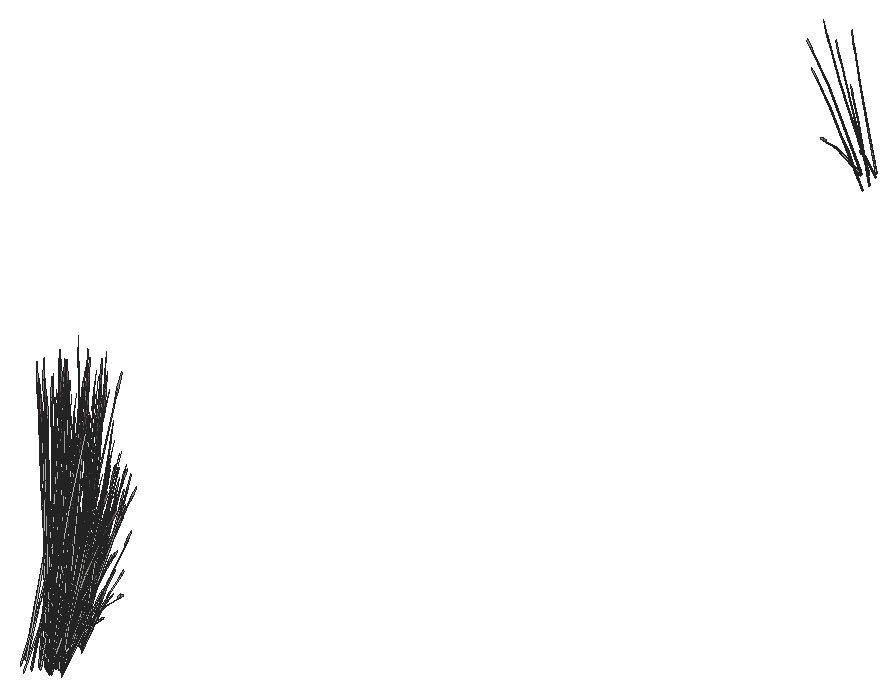
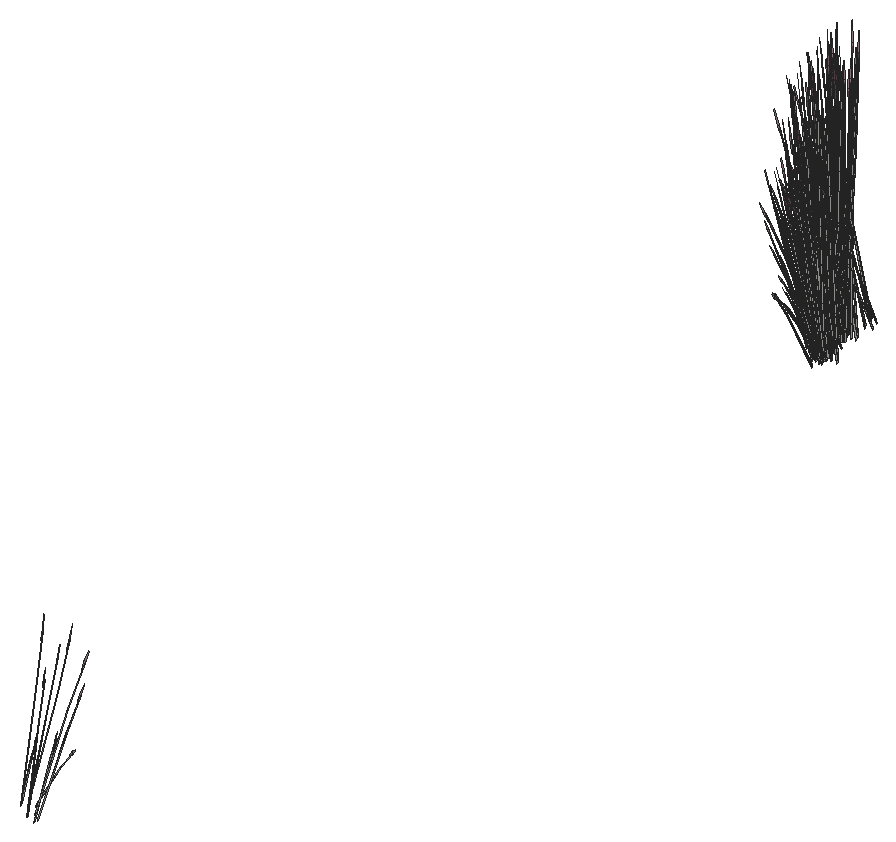
# SketchUp Ruby script. Lengths in inches.
U = 1.inch
M = Sketchup.active_model
def pt(a) = Geom::Point3d.new(a.map { |v| v * U })
def face(e, loops, mat)
  f = e.add_face(loops[0].map { |a| pt(a) })
  loops[1..].each { |l| e.add_face(l.map { |a| pt(a) }).erase! }
  f.material = f.back_material = mat if mat
  f
end
# faces: each face lists its corners as indices into pts; further lists are holes
def faces(e, pts, list, mat = nil) = list.each { |f| face(e, (f[0].is_a?(Array) ? f : [f]).map { |l| l.map { |i| pts[i] } }, mat) }
# xy, xz, yz: faces in a plane at the given z, y or x. An outline is a flat list of corners, or four numbers for a rectangle; further outlines are holes
def ring(l) = l.size == 4 ? [[l[0], l[1]], [l[2], l[1]], [l[2], l[3]], [l[0], l[3]]] : l.each_slice(2).to_a
def flat(e, list, mat, &to3) = list.each { |f| face(e, (f[0].is_a?(Array) ? f : [f]).map { |l| ring(l).map { |u, v| to3.(u, v) } }, mat) }
def xy(e, z, list, mat = nil) = flat(e, list, mat) { |x, y| [x, y, z] }
def xz(e, y, list, mat = nil) = flat(e, list, mat) { |x, z| [x, y, z] }
def yz(e, x, list, mat = nil) = flat(e, list, mat) { |y, z| [x, y, z] }
def lines(e, pts, list) = list.each { |a, b| e.add_line(pt(pts[a]), pt(pts[b])) }
# prism: a flat outline (further loops are holes) pulled along v
def prism(e, loops, v, mat = nil)
  f = face(e, loops, mat); d = Geom::Vector3d.new(v.map { |x| x * U })
  f.pushpull(f.normal.samedirection?(d) ? d.length : -d.length)
end
def box(e, o, s, mat = nil) = prism(e, [[o, [o[0] + s[0], o[1], o[2]], [o[0] + s[0], o[1] + s[1], o[2]], [o[0], o[1] + s[1], o[2]]]], [0, 0, s[2]], mat)
def at(x, y, z, deg = 0) = Geom::Transformation.translation(pt([x, y, z])) * Geom::Transformation.rotation(ORIGIN, Z_AXIS, deg.degrees)
def axes(o, x, y, z) = Geom::Transformation.new([*x, 0, *y, 0, *z, 0, *pt(o).to_a, 1])
def part(name) = M.definitions.add(name)
# library, detail: a bought-in or finely detailed component or shape, given as its bounding box
def library(name, o, s) = part(name).tap { |d| box(d.entities, o, s) }
def detail(e, o, s) = box(e.add_group.entities, o, s)
def put(e, d, t, mat = nil) = e.add_instance(d, t).tap { |i| i.material = mat if mat }
def group(e, t, mat = nil) = e.add_group.tap { |g| g.transformation = t; g.material = mat if mat }.entities
root = M.entities
M.materials.add("LightPink_Translucent").color = [144, 107, 117]
M.materials["LightPink_Translucent"].alpha = 0.75
c1 = part("blade")
p = [[2.15,0.21,22],[0,0.17,0],[0.09,0.45,0],[2.18,0.31,22],[2.29,0.31,22],[0.38,0.45,0],
  [2.48,0.24,33],[2.49,0.24,33],[2.48,0.22,33]]
faces(c1.entities,p,[[0,1,2,3],[4,5,2,3],[6,3,4,7],[8,0,3,6]])
c2 = part("seeds")
p = [[0.3,-0.1,1.38],[-0.01,-0.03,1.59],[-0.01,-0.03,0.03],[0.14,-0.07,-0.07],[0.29,-0.03,3],[0.15,0.01,3.11]]
faces(c2.entities,p,[[0,1,2,3],[1,0,4,5]],"LightPink_Translucent")
c3 = part("blade with seeds")
put(c3.entities,c1,at(0,0,0))
put(c3.entities,c2,axes([2.4,0.25,30.99],[1.5799,-0.05474,1.17369],[-0.12525,1.92788,0.29478],[-0.07173,-0.02425,1.56792]))
put(root,c3,axes([410.29,64.75,-7.64],[0.13855,-0.49442,-0.47583],[0.47502,0.16947,-0.36857],[0.19125,-0.04534,0.91046]))
put(root,c3,axes([409.54,62.74,-9.79],[0.31974,-0.54466,0],[0.53494,0.30375,-0.48057],[0.12184,0.06918,1.52448]))
put(root,c3,axes([407.34,61.09,-9.52],[-0.32795,-0.01705,0.97832],[0.21658,-0.36206,0.54015],[0.12956,0.12863,0.76741]))
put(root,c3,axes([407.69,64.43,-9.8],[0.22235,0.6078,0.42607],[-0.63531,0.21135,0.16719],[0.00776,-0.11168,1.47927]))
put(root,c3,axes([406.39,61,-7.6],[-0.23243,0.34529,0.05988],[-0.331,-0.20103,0.47138],[0.10701,0.1107,0.71878]))
put(root,c3,axes([410.8,64.89,-10.15],[-0.32938,0.06523,1.31842],[-0.05243,-0.51922,0.07547],[0.2307,-0.07859,0.75023]))
put(root,c3,axes([411.4,64.43,-9.89],[-0.31706,-0.34757,-0.06041],[0.34725,-0.31847,-0.27392],[0.09839,-0.02242,0.90349]))
put(root,c3,axes([408.49,64.48,-9.95],[0,-0.62892,0],[0.63949,0,0],[0,0,1.6711]))
put(root,c3,axes([406.49,60.9,-7.59],[-0.50866,0.12474,0.447],[-0.08828,-0.48932,0.36857],[0.11963,0.14421,0.92496]))
put(root,c3,axes([409.27,63.03,-9.69],[-0.47863,-0.27177,0.46235],[0.28609,-0.48733,0],[0.10901,0.0619,1.46668]))
put(root,c3,axes([410.2,64.93,-7.36],[0.44939,-0.24006,-0.66157],[0.25044,0.49415,0.07984],[0.21713,-0.05613,0.93586]))
put(root,c3,axes([408.1875,64.08,-9.8],[-0.42403,0.49328,0.42607],[-0.50377,-0.43543,0.16719],[0.10223,-0.04923,1.47927]))
put(root,c3,axes([406.27,60.21,-9.59],[0.00902,-0.18018,1.33163],[0.43127,-0.20126,-0.28638],[0.13313,0.21566,0.56934]))
put(root,c3,axes([408.65,64.97,-9.86],[-0.47569,-0.46784,-0.05709],[0.47598,-0.46812,0],[-0.01661,-0.01634,1.63492]))
put(root,c3,axes([407.45,63.27,-9.7],[-0.14774,0.54019,0.16428],[-0.54062,-0.15287,0.32672],[0.09339,-0.00263,1.49371]))
put(root,c3,axes([410.14,65.03,-7.3],[-0.42502,-0.15163,0.32977],[0.12396,-0.44238,-0.42575],[0.17112,-0.04056,0.81462]))
put(root,c3,axes([407.23,63.71,-10.52],[-0.50338,0.21762,1.20058],[-0.16022,-0.62439,0.4665],[0.30911,0.01039,1.36553]))
put(root,c3,axes([408.58,63.87,-9.5625],[0.09866,-0.48509,0.13483],[0.48202,0.0842,-0.38503],[0.08772,0.04981,1.18024]))
put(root,c3,axes([411.16,64.55,-10.61],[-0.02673,-0.08252,1.6421],[0.18538,-0.48271,-0.25086],[0.187,-0.00694,0.2797]))
put(root,c3,axes([408.375,64,-9.47],[-0.30722,-0.45622,0.41661],[0.46535,-0.32126,-0.2005],[0.09942,0.05645,1.33761]))
put(root,c3,axes([405.81,59.86,-8.39],[-0.1169,-0.17452,1.59586],[0.54019,-0.14692,0.12904],[0.12209,0.27397,0.68222]))
put(root,c3,axes([407.4,66.06,-9.7],[0.54955,-0.14427,0.16428],[0.1357,0.53689,0.32672],[-0.04901,-0.07823,1.49371]))
put(root,c3,axes([408.53,64.03,-9.52],[0.51635,-0.36087,-0.27094],[0.34336,0.5099,-0.46562],[0.1274,0.05178,1.4872]))
put(root,c3,axes([410.58,64.98,-7.78],[0.42502,0.15163,-0.32977],[-0.12396,0.44238,0.42575],[0.17112,-0.04056,0.81462]))
put(root,c3,axes([409.83,63.07,-10.12],[0.47863,0.27177,-0.46235],[-0.28609,0.48733,0],[0.10901,0.0619,1.46668]))
put(root,c3,axes([408.92,64.62,-9.95],[0.57217,0,0],[0,0.56272,0],[0,0,1.66132]))
put(root,c3,axes([409.09,63.3,-9.7],[-0.54955,0.14427,0.16428],[-0.1357,-0.53689,0.32672],[0.04901,0.07823,1.49371]))
put(root,c3,axes([409.43,64.43,-8.39],[-0.21212,0.01231,1.59586],[0.14072,-0.53355,0.12904],[0.3023,0.033,0.68222]))
put(root,c3,axes([409.7,63.27,-10.11],[0.12013,0.47362,-0.28847],[-0.47712,0.13449,0.28847],[0.09619,0.05462,1.29413]))
put(root,c3,axes([410.52,65.17,-7.6],[0.18783,0.37061,0.05988],[-0.34252,0.1814,0.47138],[0.15099,-0.03579,0.71878]))
put(root,c3,axes([408.74,64.33,-9.78],[-0.64638,-0.11452,0.45814],[0.13155,-0.64678,0.17978],[0.09446,0.06245,1.59061]))
put(root,c3,axes([410.49,65.03,-7.59],[-0.14449,0.4956,0.447],[-0.47502,-0.16947,0.36857],[0.1868,-0.02978,0.92496]))
put(root,c3,axes([408.22,65.93,-9.95],[-0.16686,-0.46861,0],[0.47648,-0.16411,0],[0,0,1.4375]))
put(root,c3,axes([408.85,65.86,-9.97],[0.53691,-0.18442,-0.17877],[0.18866,0.53125,0.00007],[0.05927,-0.02038,1.61933]))
put(root,c3,axes([409.03,66.09,-9.7],[0.14774,-0.54019,0.16428],[0.54062,0.15287,0.32672],[-0.09339,0.00263,1.49371]))
put(root,c3,axes([408.91,64.86,-9.9375],[0.35699,0.35109,0],[-0.35699,0.35109,0],[0,0,1.57621]))
put(root,c3,axes([409.88,64.71,-9.7],[-0.40181,-0.39593,0.16428],[0.40492,-0.38402,0.32672],[-0.04438,0.08086,1.49371]))
put(root,c3,axes([409.13,64.11,-10.08],[0.53199,0.08911,-0.58063],[-0.11226,0.54969,-0.15239],[0.15876,0.06661,1.28164]))
put(root,c3,axes([411.49,65.07,-9.42],[-0.31598,0.08973,1.06958],[0.14873,-0.37085,0.78586],[0.16763,0.02538,0.23558]))
put(root,c3,axes([408.11,66.14,-9.95],[-0.51557,-0.24403,0],[0.24813,-0.50705,0],[0,0,1.51513]))
put(root,c3,axes([408.91,64.45,-9.47],[0.24813,-0.48978,0.41661],[0.51557,0.23571,-0.2005],[0,0.1129,1.33761]))
put(root,c3,axes([411.34,66.64,-7.62],[-0.04624,-0.04758,1.65179],[0.10116,-0.51007,-0.15608],[0.18215,-0.03259,0.29231]))
put(root,c3,axes([408.8125,64.73,-9.87],[0,0.62861,-0.05249],[-0.63949,0,0],[0,0.01975,1.67027]))
put(root,c3,axes([408.86,64.28,-9.94],[0.30722,0.45622,-0.41661],[-0.46535,0.32126,0.2005],[0.09942,0.05645,1.33761]))
put(root,c3,axes([410.9375,66.21,-8.34],[-0.09788,-0.45691,-0.03251],[0.46264,-0.10504,-0.14742],[0.09661,0.02897,0.48626]))
put(root,c3,axes([409.74,66.2,-7.3125],[0.02738,-0.55277,-0.11324],[0.51847,0.01511,-0.62851],[0.19968,0.0384,0.95501]))
put(root,c3,axes([410.21,64.72,-9.69],[0,-0.54355,0.46235],[0.57217,0,0],[0,0.1238,1.46668]))
put(root,c3,axes([406.62,70.43,-9.59],[-0.14537,0.11002,1.33163],[-0.43536,-0.19256,-0.28638],[0.0807,-0.23948,0.56934]))
put(root,c3,axes([408.78,65.13,-9.47],[0.55535,-0.03355,0.41661],[0.05022,0.55698,-0.2005],[-0.09942,0.05645,1.33761]))
put(root,c3,axes([409.12,64.5625,-9.5625],[0.47648,-0.15851,0.13483],[0.16686,0.45265,-0.38503],[0,0.09962,1.18024]))
put(root,c3,axes([409.66,65.98,-7.3],[-0.29098,-0.34031,0.32977],[0.33226,-0.32215,-0.42575],[0.16881,0.04902,0.81462]))
put(root,c3,axes([410.89,65.66,-9.59],[-0.12317,-0.13368,1.33163],[0.16025,-0.44223,-0.28638],[0.24919,0.05991,0.56934]))
put(root,c3,axes([408.69,66.15,-9.95],[0.51557,0.24403,0],[-0.24813,0.50705,0],[0,0,1.62917]))
put(root,c3,axes([406.97,71.25,-7.36],[0.01331,-0.50278,-0.66157],[0.56035,0.03377,0.07984],[0.05914,-0.213,0.93586]))
put(root,c3,axes([410.1875,65.87,-7.61],[0.10971,-0.00919,1.62908],[0.30091,-0.42228,-0.25764],[0.19514,0.05574,0.13065]))
put(root,c3,axes([407.75,70.46,-7.61],[-0.00494,-0.10818,1.62908],[-0.41695,-0.31265,-0.25764],[0.06446,-0.18952,0.13065]))
put(root,c3,axes([406.34,70.99,-8.39],[-0.09522,0.18683,1.59586],[-0.39947,-0.38663,0.12904],[0.18021,-0.24097,0.68222]))
put(root,c3,axes([408.79,65.37,-9.5625],[0.37783,0.32657,0.13483],[-0.31516,0.36844,-0.38503],[-0.08772,0.04981,1.18024]))
put(root,c3,axes([409.76,65.93,-7.36],[0.51122,0.01309,-0.66157],[-0.03434,0.5511,0.07984],[0.21658,0.05816,0.93586]))
put(root,c3,axes([406.86,71.08,-7.64],[-0.3661,-0.36521,-0.47583],[0.38674,-0.31985,-0.36857],[0.0557,-0.18556,0.91046]))
put(root,c3,axes([409.1875,66.375,-9.69],[0.47863,-0.27177,0.46235],[0.28609,0.48733,0],[-0.10901,0.0619,1.46668]))
put(root,c3,axes([408.51,65.95,-9.87],[0.22235,0.62444,-0.05599],[-0.63531,0.21881,0],[0.00776,0.02181,1.60327]))
put(root,c3,axes([410.6,64.82,-9.79],[0.63949,0,0],[0,0.60749,-0.48057],[0,0.13836,1.52448]))
put(root,c3,axes([410.34,65.13,-9.95],[-0.63917,-0.00435,-0.04634],[0,-0.60749,0.46507],[-0.02009,0.13829,1.47457]))
put(root,c3,axes([408.96,64.6,-9.52],[0.57594,0.25935,-0.27094],[-0.27732,0.5474,-0.46562],[0.0181,0.1344,1.4872]))
put(root,c3,axes([407.2,70.94,-7.78],[0.34603,-0.28618,-0.32977],[0.32756,0.32677,0.42575],[0.04984,-0.16603,0.81462]))
put(root,c3,axes([410.07,66.16,-7.78],[0.29098,0.34031,-0.32977],[-0.33226,0.32215,0.42575],[0.16881,0.04902,0.81462]))
put(root,c3,axes([410.21,65.22,-10.11],[-0.35699,0.33913,-0.28847],[-0.35699,-0.33913,0.28847],[0,0.10923,1.29413]))
put(root,c3,axes([409.92,66.29,-7.6],[-0.02575,0.41332,0.05988],[-0.38885,-0.01133,0.47138],[0.14895,0.04325,0.71878]))
put(root,c3,axes([408.9,65.01,-9.94],[-0.24813,0.48978,-0.41661],[-0.51557,-0.23571,0.2005],[0,0.1129,1.33761]))
put(root,c3,axes([409.96,66.16,-7.59],[-0.37709,0.35815,0.447],[-0.32522,-0.38035,0.36857],[0.17692,0.06607,0.92496]))
put(root,c3,axes([408.76,66.57,-7.3],[-0.07899,-0.43781,0.32977],[0.45153,-0.11561,-0.42575],[0.12128,0.12546,0.81462]))
put(root,c3,axes([408.91,66.41,-9.83],[0.64025,0.17667,0.2864],[-0.16018,0.63149,-0.33981],[-0.10597,0.07904,1.53541]))
put(root,c3,axes([410.45,65.23,-10.12],[0,0.54355,-0.46235],[-0.57217,0,0],[0,0.1238,1.46668]))
put(root,c3,axes([407.64,70.77,-10.61],[-0.07655,-0.04282,1.6421],[-0.19662,-0.47839,-0.25086],[0.13264,-0.12982,0.2797]))
put(root,c3,axes([409.02,65.29,-8.39],[-0.18996,-0.09365,1.59586],[0.39312,-0.39287,0.12904],[0.24502,0.17723,0.68222]))
put(root,c3,axes([409.0625,64.06,-7.83],[-0.44191,-0.28242,1.28769],[0.46662,-0.43971,0.5556],[0.14258,0.26499,1.24467]))
put(root,c3,axes([407.2,71.06,-7.59],[0.36417,0.37086,0.447],[-0.38674,0.31985,0.36857],[0.06718,-0.174,0.92496]))
put(root,c3,axes([409.73,66.35,-9.42],[-0.28795,-0.15629,1.06958],[0.37181,-0.1588,0.78586],[0.10029,0.13452,0.23558]))
put(root,c3,axes([407.34,71.09,-7.6],[0.42027,0.02533,0.05988],[-0.01152,0.38243,0.47138],[0.04398,-0.14649,0.71878]))
put(root,c3,axes([408.72,66.8,-7.3125],[0.30474,-0.46525,-0.11324],[0.44133,0.26804,-0.62851],[0.15341,0.13145,0.95501]))
put(root,c3,axes([407.02,71.35,-7.3],[-0.34603,0.28618,0.32977],[-0.32756,-0.32677,-0.42575],[0.04984,-0.16603,0.81462]))
put(root,c3,axes([407.63,72.12,-7.36],[0.26714,-0.42887,-0.66157],[0.46811,0.30479,0.07984],[0.1595,-0.15539,0.93586]))
put(root,c3,axes([407.62,71.92,-7.64],[-0.13138,-0.49631,-0.47583],[0.49754,-0.08682,-0.36857],[0.14258,-0.13331,0.91046]))
put(root,c3,axes([409.3,66.75,-9.79],[0.31974,0.54466,0],[-0.53494,0.30375,-0.48057],[-0.12184,0.06918,1.52448]))
put(root,c3,axes([408.32,67.1875,-7.62],[0.00151,-0.06581,1.65179],[0.43826,-0.29033,-0.15608],[0.15223,0.10363,0.29231]))
put(root,c3,axes([409.81,66.94,-10.61],[0.03726,-0.07847,1.6421],[0.46909,-0.23111,-0.25086],[0.14221,0.11962,0.2797]))
put(root,c3,axes([409.1875,65.15,-10.05],[0.18752,0.49766,-0.6445],[-0.54017,0.17923,-0.16915],[0.02073,0.16852,1.42262]))
put(root,c3,axes([407.85,72.28,-7.3125],[-0.47307,-0.29971,-0.11324],[0.27254,-0.43404,-0.62851],[0.13365,-0.15087,0.95501]))
put(root,c3,axes([409.08,66.57,-7.64],[0.50465,-0.12921,-0.47583],[0.08828,0.48932,-0.36857],[0.13555,0.14022,0.91046]))
put(root,c3,axes([407.68,66.64,-7.3],[0.15418,-0.41799,0.32977],[0.44981,0.12192,-0.42575],[0.04124,0.16829,0.81462]))
put(root,c3,axes([409.77,67.07,-9.52],[-0.32795,-0.01705,0.97832],[0.21658,-0.36206,0.54015],[0.12956,0.12863,0.76741]))
put(root,c3,axes([405.18,70.79,-10.12],[0.47863,-0.27177,-0.46235],[0.28609,0.48733,0],[0.10901,-0.0619,1.46668]))
put(root,c3,axes([408.02,71.73,-9.59],[-0.1827,-0.0161,1.33163],[-0.18717,-0.43188,-0.28638],[0.22444,-0.12218,0.56934]))
put(root,c3,axes([409.02,72.15,-7.62],[-0.0668,-0.00413,1.65179],[-0.27738,-0.44233,-0.15608],[0.11139,-0.14544,0.29231]))
put(root,c3,axes([408.83,66.97,-7.6],[-0.23243,0.34529,0.05988],[-0.331,-0.20103,0.47138],[0.10701,0.1107,0.71878]))
put(root,c3,axes([408.28,68.13,-6.74],[0.35341,-0.31182,-0.06041],[0.32382,0.34152,-0.27392],[0.0228,0.09677,0.90349]))
put(root,c3,axes([405.75,71.9,-10.08],[0.34446,-0.40855,-0.58063],[0.42791,0.37046,-0.15239],[0.13803,-0.10191,1.28164]))
put(root,c3,axes([408.93,66.875,-7.59],[-0.50866,0.12474,0.447],[-0.08828,-0.48932,0.36857],[0.11963,0.14421,0.92496]))
put(root,c3,axes([408.23,70.93,-9.42],[-0.17034,0.27669,1.06958],[-0.14642,-0.37174,0.78586],[0.14069,-0.09315,0.23558]))
put(root,c3,axes([408.7,66.1875,-9.59],[0.00902,-0.18018,1.33163],[0.43127,-0.20126,-0.28638],[0.13313,0.21566,0.56934]))
put(root,c3,axes([407.99,71.97,-7.78],[0.44516,-0.07768,-0.32977],[0.11755,0.44407,0.42575],[0.12757,-0.11927,0.81462]))
put(root,c3,axes([407.54,67.02,-7.6],[-0.37684,0.18473,0.05988],[-0.18445,-0.33686,0.47138],[0.03639,0.14849,0.71878]))
put(root,c3,axes([407.53,66.82,-7.3125],[0.50045,-0.25306,-0.11324],[0.24593,0.44915,-0.62851],[0.06603,0.18927,0.95501]))
put(root,c3,axes([405.375,72.375,-9.52],[-0.05959,-0.62022,-0.27094],[0.62068,-0.0375,-0.46562],[0.1093,-0.08261,1.4872]))
put(root,c3,axes([407.67,66.99,-7.28],[-0.50393,-0.1421,0.49617],[0.17232,-0.46717,0.40911],[0.03028,0.18372,1.0267]))
put(root,c3,axes([407.625,72.23,-7.3],[-0.44516,0.07768,0.32977],[-0.11755,-0.44407,-0.42575],[0.12757,-0.11927,0.81462]))
put(root,c3,axes([407.62,66.92,-10.61],[0.08277,-0.02958,1.6421],[0.49786,0.16279,-0.25086],[0.01456,0.18348,0.2797]))
put(root,c3,axes([405.29,71,-10.11],[0.47712,0.13449,-0.28847],[-0.12013,0.47362,0.28847],[0.09619,-0.05462,1.29413]))
put(root,c3,axes([407.96,66.8,-7.64],[0.50273,0.13626,-0.47583],[-0.17232,0.46717,-0.36857],[0.0461,0.18809,0.91046]))
put(root,c3,axes([408.24,65.83,-8.39],[-0.1169,-0.17452,1.59586],[0.54019,-0.14692,0.12904],[0.12209,0.27397,0.68222]))
put(root,c3,axes([408.03,72.16,-7.6],[0.35109,0.22859,0.05988],[-0.2044,0.32553,0.47138],[0.11256,-0.10524,0.71878]))
put(root,c3,axes([407.93,72.07,-7.59],[0.12683,0.50025,0.447],[-0.49754,0.08682,0.36857],[0.14663,-0.11765,0.92496]))
put(root,c3,axes([409.27,72.67,-7.61],[0.07097,-0.08279,1.62908],[-0.09083,-0.50786,-0.25764],[0.17806,-0.09629,0.13065]))
put(root,c3,axes([407.73,67.08,-7.78],[-0.15418,0.41799,-0.32977],[-0.44981,-0.12192,0.42575],[0.04124,0.16829,0.81462]))
put(root,c3,axes([407.77,66.71,-7.36],[0.24409,0.44196,-0.66157],[-0.50245,0.2463,0.07984],[0.05708,0.21354,0.93586]))
put(root,c3,axes([407.41,67.82,-7.61],[0.06483,0.08753,1.62908],[0.52315,0.03439,-0.25764],[0.05261,0.19303,0.13065]))
put(root,c3,axes([407.875,73.44,-7.3125],[-0.25732,-0.49218,-0.11324],[0.45669,-0.24187,-0.62851],[0.19245,-0.06494,0.95501]))
put(root,c3,axes([407.85,73.02,-7.64],[0.13855,-0.49442,-0.47583],[0.47502,0.16947,-0.36857],[0.19125,-0.04534,0.91046]))
put(root,c3,axes([407.1,71.01,-9.79],[0.31974,-0.54466,0],[0.53494,0.30375,-0.48057],[0.12184,0.06918,1.52448]))
put(root,c3,axes([408.36,73.16,-10.15],[-0.32938,0.06523,1.31842],[-0.05243,-0.51922,0.07547],[0.2307,-0.07859,0.75023]))
put(root,c3,axes([408.96,72.7,-9.89],[-0.31706,-0.34757,-0.06041],[0.34725,-0.31847,-0.27392],[0.09839,-0.02242,0.90349]))
put(root,c3,axes([406.82,71.29,-9.69],[-0.47863,-0.27177,0.46235],[0.28609,-0.48733,0],[0.10901,0.0619,1.46668]))
put(root,c3,axes([407.76,73.2,-7.36],[0.44939,-0.24006,-0.66157],[0.25044,0.49415,0.07984],[0.21713,-0.05613,0.93586]))
put(root,c3,axes([407.7,73.3,-7.3],[-0.42502,-0.15163,0.32977],[0.12396,-0.44238,-0.42575],[0.17112,-0.04056,0.81462]))
put(root,c3,axes([404.79,71.97,-10.52],[-0.50338,0.21762,1.20058],[-0.16022,-0.62439,0.4665],[0.30911,0.01039,1.36553]))
put(root,c3,axes([406.14,72.14,-9.5625],[0.09866,-0.48509,0.13483],[0.48202,0.0842,-0.38503],[0.08772,0.04981,1.18024]))
put(root,c3,axes([408.72,72.82,-10.61],[-0.02673,-0.08252,1.6421],[0.18538,-0.48271,-0.25086],[0.187,-0.00694,0.2797]))
put(root,c3,axes([405.93,72.27,-9.47],[-0.30722,-0.45622,0.41661],[0.46535,-0.32126,-0.2005],[0.09942,0.05645,1.33761]))
put(root,c3,axes([406.09,72.3,-9.52],[0.51635,-0.36087,-0.27094],[0.34336,0.5099,-0.46562],[0.1274,0.05178,1.4872]))
put(root,c3,axes([408.14,73.25,-7.78],[0.42502,0.15163,-0.32977],[-0.12396,0.44238,0.42575],[0.17112,-0.04056,0.81462]))
put(root,c3,axes([407.39,71.34,-10.12],[0.47863,0.27177,-0.46235],[-0.28609,0.48733,0],[0.10901,0.0619,1.46668]))
put(root,c3,axes([406.48,72.89,-9.95],[0.57217,0,0],[0,0.56272,0],[0,0,1.66132]))
put(root,c3,axes([406.98,72.7,-8.39],[-0.21212,0.01231,1.59586],[0.14072,-0.53355,0.12904],[0.3023,0.033,0.68222]))
put(root,c3,axes([407.26,71.54,-10.11],[0.12013,0.47362,-0.28847],[-0.47712,0.13449,0.28847],[0.09619,0.05462,1.29413]))
put(root,c3,axes([408.08,73.43,-7.6],[0.18783,0.37061,0.05988],[-0.34252,0.1814,0.47138],[0.15099,-0.03579,0.71878]))
put(root,c3,axes([408.04,73.3,-7.59],[-0.14449,0.4956,0.447],[-0.47502,-0.16947,0.36857],[0.1868,-0.02978,0.92496]))
put(root,c3,axes([406.41,74.13,-9.97],[0.53691,-0.18442,-0.17877],[0.18866,0.53125,0.00007],[0.05927,-0.02038,1.61933]))
put(root,c3,axes([406.69,72.38,-10.08],[0.53199,0.08911,-0.58063],[-0.11226,0.54969,-0.15239],[0.15876,0.06661,1.28164]))
put(root,c3,axes([409.04,73.34,-9.42],[-0.31598,0.08973,1.06958],[0.14873,-0.37085,0.78586],[0.16763,0.02538,0.23558]))
put(root,c3,axes([408.9,74.91,-7.62],[-0.04624,-0.04758,1.65179],[0.10116,-0.51007,-0.15608],[0.18215,-0.03259,0.29231]))
put(root,c3,axes([406.42,72.55,-9.94],[0.30722,0.45622,-0.41661],[-0.46535,0.32126,0.2005],[0.09942,0.05645,1.33761]))
put(root,c3,axes([408.5,74.48,-8.34],[-0.09788,-0.45691,-0.03251],[0.46264,-0.10504,-0.14742],[0.09661,0.02897,0.48626]))
put(root,c3,axes([407.3,74.47,-7.3125],[0.02738,-0.55277,-0.11324],[0.51847,0.01511,-0.62851],[0.19968,0.0384,0.95501]))
put(root,c3,axes([407.77,72.99,-9.69],[0,-0.54355,0.46235],[0.57217,0,0],[0,0.1238,1.46668]))
put(root,c3,axes([406.68,72.83,-9.5625],[0.47648,-0.15851,0.13483],[0.16686,0.45265,-0.38503],[0,0.09962,1.18024]))
put(root,c3,axes([407.22,74.25,-7.3],[-0.29098,-0.34031,0.32977],[0.33226,-0.32215,-0.42575],[0.16881,0.04902,0.81462]))
put(root,c3,axes([408.45,73.93,-9.59],[-0.12317,-0.13368,1.33163],[0.16025,-0.44223,-0.28638],[0.24919,0.05991,0.56934]))
put(root,c3,axes([407.75,74.14,-7.61],[0.10971,-0.00919,1.62908],[0.30091,-0.42228,-0.25764],[0.19514,0.05574,0.13065]))
put(root,c3,axes([407.32,74.2,-7.36],[0.51122,0.01309,-0.66157],[-0.03434,0.5511,0.07984],[0.21658,0.05816,0.93586]))
put(root,c3,axes([408.16,73.08,-9.79],[0.63949,0,0],[0,0.60749,-0.48057],[0,0.13836,1.52448]))
put(root,c3,axes([406.52,72.87,-9.52],[0.57594,0.25935,-0.27094],[-0.27732,0.5474,-0.46562],[0.0181,0.1344,1.4872]))
put(root,c3,axes([407.63,74.43,-7.78],[0.29098,0.34031,-0.32977],[-0.33226,0.32215,0.42575],[0.16881,0.04902,0.81462]))
put(root,c3,axes([407.48,74.56,-7.6],[-0.02575,0.41332,0.05988],[-0.38885,-0.01133,0.47138],[0.14895,0.04325,0.71878]))
put(root,c3,axes([407.52,74.43,-7.59],[-0.37709,0.35815,0.447],[-0.32522,-0.38035,0.36857],[0.17692,0.06607,0.92496]))
put(root,c3,axes([406.32,74.84,-7.3],[-0.07899,-0.43781,0.32977],[0.45153,-0.11561,-0.42575],[0.12128,0.12546,0.81462]))
put(root,c3,axes([408.01,73.5,-10.12],[0,0.54355,-0.46235],[-0.57217,0,0],[0,0.1238,1.46668]))
put(root,c3,axes([406.58,73.56,-8.39],[-0.18996,-0.09365,1.59586],[0.39312,-0.39287,0.12904],[0.24502,0.17723,0.68222]))
put(root,c3,axes([406.62,72.32,-7.83],[-0.44191,-0.28242,1.28769],[0.46662,-0.43971,0.5556],[0.14258,0.26499,1.24467]))
put(root,c3,axes([407.29,74.62,-9.42],[-0.28795,-0.15629,1.06958],[0.37181,-0.1588,0.78586],[0.10029,0.13452,0.23558]))
put(root,c3,axes([406.28,75.07,-7.3125],[0.30474,-0.46525,-0.11324],[0.44133,0.26804,-0.62851],[0.15341,0.13145,0.95501]))
put(root,c3,axes([405.875,75.45,-7.62],[0.00151,-0.06581,1.65179],[0.43826,-0.29033,-0.15608],[0.15223,0.10363,0.29231]))
put(root,c3,axes([407.37,75.2,-10.61],[0.03726,-0.07847,1.6421],[0.46909,-0.23111,-0.25086],[0.14221,0.11962,0.2797]))
put(root,c3,axes([406.75,73.42,-10.05],[0.18752,0.49766,-0.6445],[-0.54017,0.17923,-0.16915],[0.02073,0.16852,1.42262]))
put(root,c3,axes([406.64,74.84,-7.64],[0.50465,-0.12921,-0.47583],[0.08828,0.48932,-0.36857],[0.13555,0.14022,0.91046]))
put(root,c3,axes([407.33,75.33,-9.52],[-0.32795,-0.01705,0.97832],[0.21658,-0.36206,0.54015],[0.12956,0.12863,0.76741]))
put(root,c3,axes([406.39,75.24,-7.6],[-0.23243,0.34529,0.05988],[-0.331,-0.20103,0.47138],[0.10701,0.1107,0.71878]))
put(root,c3,axes([406.49,75.14,-7.59],[-0.50866,0.12474,0.447],[-0.08828,-0.48932,0.36857],[0.11963,0.14421,0.92496]))
put(root,c3,axes([406.26,74.46,-9.59],[0.00902,-0.18018,1.33163],[0.43127,-0.20126,-0.28638],[0.13313,0.21566,0.56934]))
put(root,c3,axes([405.8,74.1,-8.39],[-0.1169,-0.17452,1.59586],[0.54019,-0.14692,0.12904],[0.12209,0.27397,0.68222]))
put(root,c3,axes([411.21,278.68,-8.39],[0.1169,0.17452,1.59586],[-0.54019,0.14692,0.12904],[-0.12209,-0.27397,0.68222]))
put(root,c3,axes([412.1,277.52,-7.61],[-0.07822,-0.07621,1.62908],[-0.52201,0.04832,-0.25764],[-0.08331,-0.18228,0.13065]))
put(root,c3,axes([413.31,278.42,-9.59],[-0.14537,0.11002,1.33163],[-0.43536,-0.19256,-0.28638],[0.0807,-0.23948,0.56934]))
put(root,c3,axes([412.64,278.81,-7.36],[-0.24409,-0.44196,-0.66157],[0.50245,-0.2463,0.07984],[-0.05708,-0.21354,0.93586]))
put(root,c3,axes([411.06,278.22,-9.59],[-0.03097,0.17781,1.33163],[-0.45273,0.14885,-0.28638],[-0.10583,-0.22982,0.56934]))
put(root,c3,axes([412.22,277.83,-10.61],[-0.08578,0.01958,1.6421],[-0.47437,-0.22044,-0.25086],[0.00796,-0.18387,0.2797]))
put(root,c3,axes([413.66,279.24,-7.36],[0.01331,-0.50278,-0.66157],[0.56035,0.03377,0.07984],[0.05914,-0.213,0.93586]))
put(root,c3,axes([414.44,278.45,-7.61],[-0.00494,-0.10818,1.62908],[-0.41695,-0.31265,-0.25764],[0.06446,-0.18952,0.13065]))
put(root,c3,axes([412.69,278.43,-7.78],[0.15418,-0.41799,-0.32977],[0.44981,0.12192,0.42575],[-0.04124,-0.16829,0.81462]))
